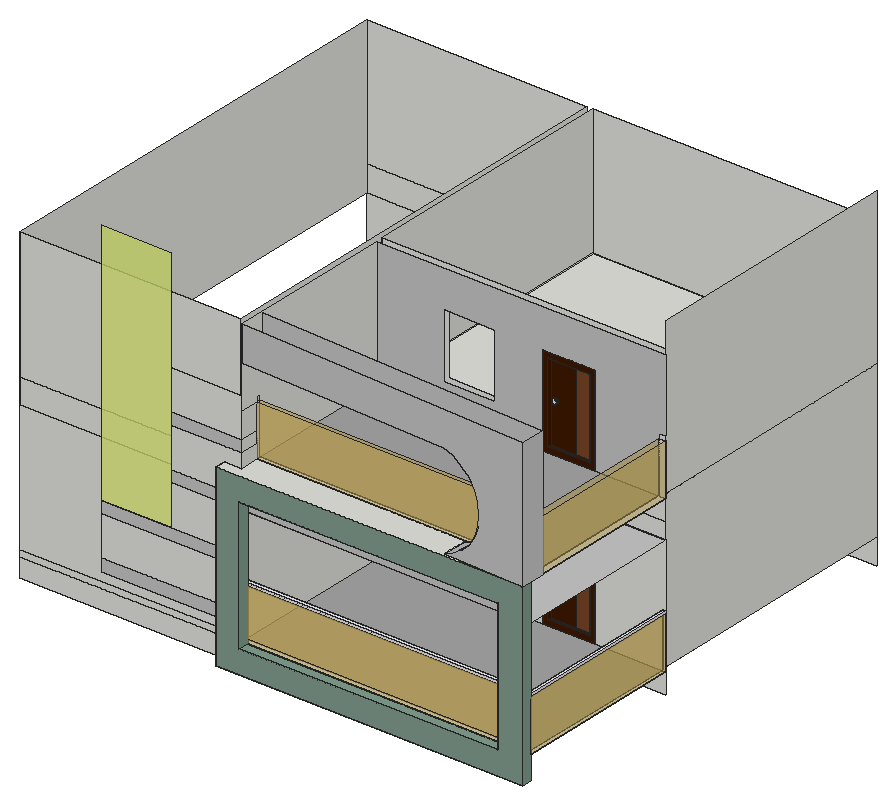
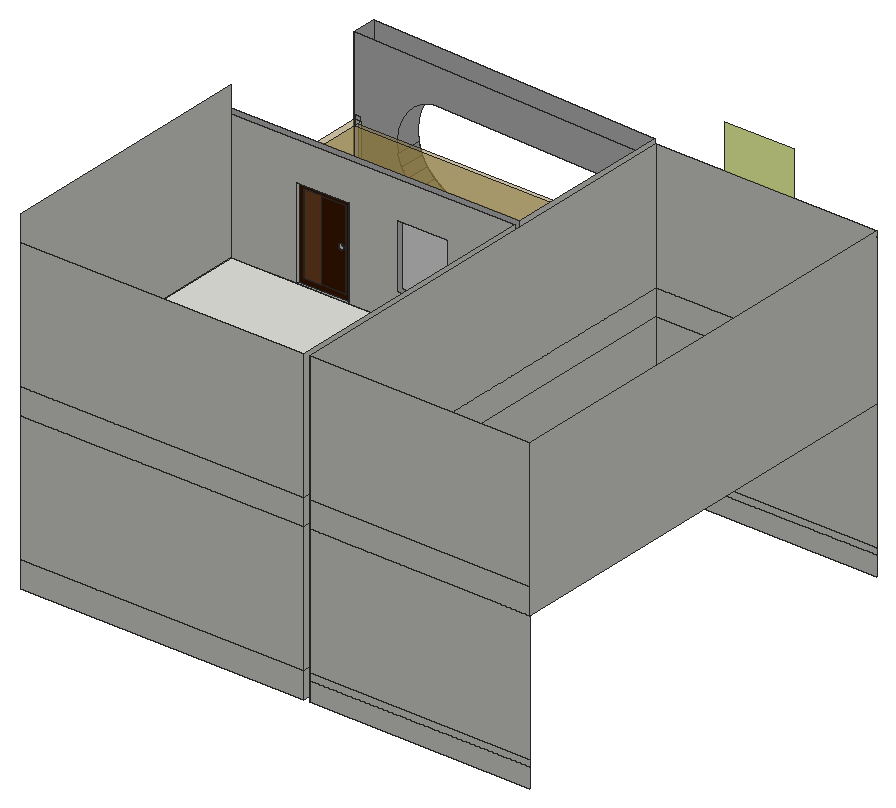
# SketchUp Ruby script. Lengths in inches.
U = 1.inch
M = Sketchup.active_model
def pt(a) = Geom::Point3d.new(a.map { |v| v * U })
def face(e, loops, mat)
  f = e.add_face(loops[0].map { |a| pt(a) })
  loops[1..].each { |l| e.add_face(l.map { |a| pt(a) }).erase! }
  f.material = f.back_material = mat if mat
  f
end
# faces: each face lists its corners as indices into pts; further lists are holes
def faces(e, pts, list, mat = nil) = list.each { |f| face(e, (f[0].is_a?(Array) ? f : [f]).map { |l| l.map { |i| pts[i] } }, mat) }
# xy, xz, yz: faces in a plane at the given z, y or x. An outline is a flat list of corners, or four numbers for a rectangle; further outlines are holes
def ring(l) = l.size == 4 ? [[l[0], l[1]], [l[2], l[1]], [l[2], l[3]], [l[0], l[3]]] : l.each_slice(2).to_a
def flat(e, list, mat, &to3) = list.each { |f| face(e, (f[0].is_a?(Array) ? f : [f]).map { |l| ring(l).map { |u, v| to3.(u, v) } }, mat) }
def xy(e, z, list, mat = nil) = flat(e, list, mat) { |x, y| [x, y, z] }
def xz(e, y, list, mat = nil) = flat(e, list, mat) { |x, z| [x, y, z] }
def yz(e, x, list, mat = nil) = flat(e, list, mat) { |y, z| [x, y, z] }
def lines(e, pts, list) = list.each { |a, b| e.add_line(pt(pts[a]), pt(pts[b])) }
# prism: a flat outline (further loops are holes) pulled along v
def prism(e, loops, v, mat = nil)
  f = face(e, loops, mat); d = Geom::Vector3d.new(v.map { |x| x * U })
  f.pushpull(f.normal.samedirection?(d) ? d.length : -d.length)
end
def box(e, o, s, mat = nil) = prism(e, [[o, [o[0] + s[0], o[1], o[2]], [o[0] + s[0], o[1] + s[1], o[2]], [o[0], o[1] + s[1], o[2]]]], [0, 0, s[2]], mat)
def at(x, y, z, deg = 0) = Geom::Transformation.translation(pt([x, y, z])) * Geom::Transformation.rotation(ORIGIN, Z_AXIS, deg.degrees)
def axes(o, x, y, z) = Geom::Transformation.new([*x, 0, *y, 0, *z, 0, *pt(o).to_a, 1])
def part(name) = M.definitions.add(name)
# library, detail: a bought-in or finely detailed component or shape, given as its bounding box
def library(name, o, s) = part(name).tap { |d| box(d.entities, o, s) }
def detail(e, o, s) = box(e.add_group.entities, o, s)
def put(e, d, t, mat = nil) = e.add_instance(d, t).tap { |i| i.material = mat if mat }
def group(e, t, mat = nil) = e.add_group.tap { |g| g.transformation = t; g.material = mat if mat }.entities
root = M.entities
M.materials.add("[Color B08]").color = [62, 25, 0]
M.materials.add("[Color H08]").color = [130, 158, 143]
M.materials.add("[Color M02]").color = [198, 198, 198]
M.materials.add("[Metal Silver]").color = [234, 233, 238]
M.materials.add("[Stone Vein Gray]").color = [166, 165, 165]
M.materials.add("[Translucent Glass Blue]").color = [201, 149, 0]
M.materials["[Translucent Glass Blue]"].alpha = 0.5
M.materials.add("[Translucent Glass Blue]1").color = [221, 188, 93]
M.materials["[Translucent Glass Blue]1"].alpha = 0.5
M.materials.add("[Translucent Glass Corrugated]").color = [233, 249, 123]
M.materials["[Translucent Glass Corrugated]"].alpha = 0.8
M.materials.add("[Wood Veneer 01]").color = [120, 70, 37]
c1 = part("Group\#1")
xy(c1.entities,0,[[0,0,48,3.5]])
xy(c1.entities,4.73,[[4.73,0,28,3.5],[28,0,43.27,3.5]],"[Color B08]")
xy(c1.entities,79.27,[[4.73,0,28,3.5],[28,0,43.27,3.5]])
xy(c1.entities,84,[[0,0,48,3.5]],"[Color B08]")
xz(c1.entities,0,[[[0,0,48,84],[4.73,4.73,43.27,79.27]]],"[Color B08]")
xz(c1.entities,1.8125,[[8.85,40.5625,9.49,40.61,10.09,40.82,10.62,41.17,11.03,41.66,11.31,42.23,11.43,42.85,11.38,43.49,11.17,44.09,10.82,44.62,10.33,45.03,9.76,45.31,9.14,45.43,8.5,45.38,7.9,45.17,7.375,44.81,6.96,44.33,6.68,43.76,6.5625,43.14,6.61,42.5,6.82,41.9,7.17,41.375,7.66,40.96,8.23,40.68]],"[Metal Silver]")
xz(c1.entities,3.5,[[[0,0,48,84],[4.73,4.73,43.27,79.27]],[[4.73,4.73,28,79.27],[8.85,40.5625,8.23,40.68,7.66,40.96,7.17,41.375,6.82,41.9,6.61,42.5,6.5625,43.14,6.68,43.76,6.96,44.33,7.375,44.81,7.9,45.17,8.5,45.38,9.14,45.43,9.76,45.31,10.33,45.03,10.82,44.62,11.17,44.09,11.38,43.49,11.43,42.85,11.31,42.23,11.03,41.66,10.62,41.17,10.09,40.82,9.49,40.61]]],"[Color B08]")
xz(c1.entities,3.5,[[8.85,40.5625,8.23,40.68,7.66,40.96,7.17,41.375,6.82,41.9,6.61,42.5,6.5625,43.14,6.68,43.76,6.96,44.33,7.375,44.81,7.9,45.17,8.5,45.38,9.14,45.43,9.76,45.31,10.33,45.03,10.82,44.62,11.17,44.09,11.38,43.49,11.43,42.85,11.31,42.23,11.03,41.66,10.62,41.17,10.09,40.82,9.49,40.61]],"[Metal Silver]")
xz(c1.entities,3.5,[[28,4.73,43.27,79.27]],"[Wood Veneer 01]")
yz(c1.entities,0,[[0,0,3.5,84]],"[Color B08]")
yz(c1.entities,4.73,[[0,4.73,3.5,79.27]],"[Color B08]")
yz(c1.entities,43.27,[[0,4.73,3.5,79.27]],"[Color B08]")
yz(c1.entities,48,[[0,0,3.5,84]],"[Color B08]")
p = [[8.23,3.5,40.68],[8.85,3.5,40.5625],[8.85,1.8125,40.5625],[8.23,1.8125,40.68],[9.49,3.5,40.61],[9.49,1.8125,40.61],
  [10.09,3.5,40.82],[10.09,1.8125,40.82],[7.66,3.5,40.96],[7.66,1.8125,40.96],[10.62,3.5,41.17],[10.62,1.8125,41.17],
  [7.17,3.5,41.375],[7.17,1.8125,41.375],[11.03,3.5,41.66],[11.03,1.8125,41.66],[6.82,3.5,41.9],[6.82,1.8125,41.9],
  [11.31,3.5,42.23],[11.31,1.8125,42.23],[6.61,3.5,42.5],[6.61,1.8125,42.5],[11.43,3.5,42.85],[11.43,1.8125,42.85],
  [6.5625,3.5,43.14],[6.5625,1.8125,43.14],[11.38,3.5,43.49],[11.38,1.8125,43.49],[6.68,3.5,43.76],[6.68,1.8125,43.76],
  [11.17,3.5,44.09],[11.17,1.8125,44.09],[6.96,3.5,44.33],[6.96,1.8125,44.33],[10.82,3.5,44.62],[10.82,1.8125,44.62],
  [7.375,3.5,44.81],[7.375,1.8125,44.81],[10.33,3.5,45.03],[10.33,1.8125,45.03],[7.9,3.5,45.17],[7.9,1.8125,45.17],
  [9.76,3.5,45.31],[9.76,1.8125,45.31],[8.5,3.5,45.38],[8.5,1.8125,45.38],[9.14,3.5,45.43],[9.14,1.8125,45.43]]
faces(c1.entities,p,[[0,1,2,3],[1,4,5,2],[4,6,7,5],[8,0,3,9],[6,10,11,7],[12,8,9,13],[10,14,15,11],[16,12,13,17],
  [14,18,19,15],[20,16,17,21],[18,22,23,19],[24,20,21,25],[22,26,27,23],[28,24,25,29],[26,30,31,27],[32,28,29,33],
  [30,34,35,31],[36,32,33,37],[34,38,39,35],[40,36,37,41],[38,42,43,39],[44,40,41,45],[42,46,47,43],[46,44,45,47]],"[Metal Silver]")
c2 = part("Group\#2")
xy(c2.entities,0,[[0,0,48,4.9375]])
xy(c2.entities,3.28,[[23.77,0,25.1875,4.9375]])
xy(c2.entities,3.28,[[3.28,0,23.77,4.9375],[25.1875,0,44.72,4.9375]],"[Color B08]")
xy(c2.entities,56.72,[[23.77,0,25.1875,4.9375]])
xy(c2.entities,56.72,[[3.28,0,23.77,4.9375],[25.1875,0,44.72,4.9375]],"[Color B08]")
xy(c2.entities,60,[[0,0,48,4.9375]],"[Color B08]")
xz(c2.entities,0,[[[0,0,48,60],[3.28,3.28,44.72,56.72]],[23.77,3.28,25.1875,56.72]],"[Color B08]")
xz(c2.entities,4.9375,[[[0,0,48,60],[3.28,3.28,44.72,56.72]],[23.77,3.28,25.1875,56.72]],"[Color B08]")
xz(c2.entities,4.9375,[[3.28,3.28,23.77,56.72],[25.1875,3.28,44.72,56.72]],"[Translucent Glass Blue]")
yz(c2.entities,0,[[0,0,4.9375,60]],"[Color B08]")
yz(c2.entities,3.28,[[0,3.28,4.9375,56.72]],"[Color B08]")
yz(c2.entities,23.77,[[0,3.28,4.9375,56.72]],"[Color B08]")
yz(c2.entities,25.1875,[[0,3.28,4.9375,56.72]],"[Color B08]")
yz(c2.entities,44.72,[[0,3.28,4.9375,56.72]],"[Color B08]")
yz(c2.entities,48,[[0,0,4.9375,60]],"[Color B08]")
xy(root,131.51,[[269.375,132.6875,554.1875,142.1875]],"[Color H08]")
xy(root,153,[[285.75,142.1875,285.75,146.18,550.9,146.18,550.9,299.125,554.1875,299.125,554.1875,142.1875],[285.75,305.125,548.75,550.1875]])
xy(root,153,[[290.875,132.6875,531.17,142.1875]],"[Color H08]")
xy(root,153,[[285.75,146.18,550.9,146.18,550.9,299.125,487.75,299.125,487.75,305.125,439.75,305.125,439.75,299.125,285.75,299.125]],"[Stone Vein Gray]")
xy(root,182.88,[[347.8125,299.125,395.8125,305.125]])
xy(root,201,[[285.75,142.1875,285.75,146.18,550.9,146.18,550.9,299.125,554.1875,299.125,554.1875,142.1875]])
xy(root,203.625,[[285.75,142.1875,554.1875,142.1875,554.1875,299.125,550.9,299.125,550.9,146.18,285.75,146.18]],"[Metal Silver]")
xy(root,237,[[439.75,299.125,487.75,305.125]])
xy(root,242.88,[[347.8125,299.125,395.8125,305.125]])
xy(root,262.5625,[[285.75,142.1875,554.1875,299.125]],"[Color M02]")
xy(root,275.35,[[290.875,132.6875,531.17,142.1875]],"[Color H08]")
xy(root,297,[[269.375,132.6875,554.1875,132.6875,478.91,135.35,479.15,142.1875,479.42,149.6875,479.42,159.75,285.75,159.75,285.75,142.1875,269.375,142.1875],[554.1875,132.6875,554.1875,142.1875,479.15,142.1875,478.91,135.35],[554.1875,132.6875,554.1875,155.45,554.99,155.42],[479.15,142.1875,479.42,149.6875,479.71,158.09,547.7,155.68,554.1875,155.45,554.1875,142.1875],[479.42,149.6875,479.71,158.09,547.7,155.68,547.7,159.75,479.42,159.75],
  [554.1875,155.45,547.7,155.68,547.7,299.125,554.1875,299.125],[285.75,159.75,547.7,163.37],[285.75,305.125,548.75,550.1875]])
xy(root,297,[[285.75,163.37,547.7,163.37,547.7,299.125,487.75,299.125,487.75,305.125,439.75,305.125,439.75,299.125,285.75,299.125]],"[Stone Vein Gray]")
xz(root,132.6875,[[[269.375,131.51,554.1875,297],[290.875,153,531.17,275.35]]],"[Color H08]")
xz(root,142.1875,[[269.375,131.51,554.1875,153],[269.375,153,285.75,165.45],[285.75,153,290.875,201],[531.17,153,554.1875,201],[269.375,165.45,285.75,176.5],
  [155.14,176.5,269.375,213.52],[269.375,176.5,285.75,213.52],[285.75,201,290.875,203.625],[531.17,201,554.1875,203.625],[269.375,213.52,285.75,224.5625],
  [220.2,224.5625,269.375,261.58],[269.375,224.5625,285.75,261.58],[269.375,261.58,285.75,272.625],[531.17,262.5625,554.1875,276.72],[220.2,272.625,269.375,272.625,269.375,297,285.75,297,285.75,309.64,220.2,309.64],
  [220.2,320.6875,285.75,357.7]])
xz(root,142.1875,[[285.75,203.625,290.875,262.5625],[531.17,203.625,554.1875,262.5625]],"[Color H08]")
xz(root,142.1875,[[155.14,165.45,269.375,176.5],[155.14,213.52,269.375,224.5625],[220.2,261.58,269.375,272.625],[290.875,262.5625,531.17,275.35],[220.2,309.64,285.75,320.6875]],"[Color M02]")
xz(root,142.1875,[[290.875,201,531.17,203.625]],"[Metal Silver]")
xz(root,142.1875,[[290.875,153,531.17,201]],"[Translucent Glass Blue]1")
xz(root,142.1875,[[155.14,224.5625,220.2,453.83]],"[Translucent Glass Corrugated]")
xz(root,146.18,[[285.75,201,550.9,203.625]],"[Metal Silver]")
xz(root,146.18,[[285.75,153,550.9,201]],"[Translucent Glass Blue]1")
xz(root,148.1875,[[75,129,279.75,147],[75,147,279.75,153],[75,153,279.75,273],[75,273,279.75,297],[75,297,279.75,417]])
xz(root,159.75,[[285.75,297,547.7,345]],"[Translucent Glass Blue]1")
xz(root,163.37,[[285.75,297,547.7,345]],"[Translucent Glass Blue]1")
xz(root,299.125,[[[285.75,153,439.75,153,439.75,237,487.75,237,487.75,153,550.9,153,550.9,203.625,554.1875,203.625,554.1875,262.5625,285.75,262.5625],[347.8125,182.88,395.8125,242.88]],[550.9,153,554.1875,201],[550.9,201,554.1875,203.625],[547.7,297,554.1875,345]])
xz(root,299.125,[[[285.75,297,439.75,297,439.75,381,487.75,381,487.75,297,547.7,297,547.7,349.125,554.1875,349.125,554.1875,417,285.75,417],[347.4375,322.25,395.4375,382.25]]],"[Color M02]")
xz(root,305.125,[[285.75,129,548.75,153],[[285.75,153,285.75,273,548.75,273,548.75,153,487.75,153,487.75,237,439.75,237,439.75,153],[347.8125,182.88,395.8125,242.88]],[285.75,273,548.75,297],[[285.75,297,285.75,417,548.75,417,548.75,297,487.75,297,487.75,381,439.75,381,439.75,297],[347.4375,322.25,395.4375,382.25]]])
xz(root,550.1875,[[75,129,279.75,147],[285.75,129,548.75,153],[75,147,279.75,153],[75,153,279.75,273],[285.75,153,548.75,273],
  [75,273,279.75,297],[285.75,273,548.75,297],[75,297,279.75,417],[285.75,297,548.75,417]])
yz(root,75,[[148.1875,273,550.1875,417]])
yz(root,269.375,[[132.6875,131.51,142.1875,297]],"[Color H08]")
yz(root,279.75,[[148.1875,129,550.1875,147],[148.1875,147,211.54,153],[211.54,147,221.6,153],[221.6,147,550.1875,153],[148.1875,153,550.1875,273],
  [148.1875,273,550.1875,297],[148.1875,297,550.1875,417]])
yz(root,285.75,[[305.125,129,550.1875,153],[142.1875,153,146.18,201],[146.18,153,299.125,153,299.125,262.5625,142.1875,262.5625,142.1875,203.625,146.18,203.625],[305.125,153,550.1875,273],[142.1875,201,146.18,203.625],
  [305.125,273,550.1875,297],[142.1875,297,159.75,309.64],[163.37,297,299.125,297,299.125,417,142.1875,417,142.1875,345,159.75,345,159.75,349.125,163.37,349.125],[159.75,297,163.37,345],[305.125,297,550.1875,417],
  [142.1875,309.64,159.75,320.6875],[142.1875,320.6875,159.75,345]])
yz(root,290.875,[[132.6875,153,142.1875,275.35]],"[Color H08]")
yz(root,347.8125,[[299.125,182.88,305.125,242.88]])
yz(root,395.8125,[[299.125,182.88,305.125,242.88]])
yz(root,439.75,[[299.125,153,305.125,237],[299.125,297,305.125,381]])
yz(root,487.75,[[299.125,153,305.125,237],[299.125,297,305.125,381]])
yz(root,531.17,[[132.6875,153,142.1875,275.35]])
yz(root,547.7,[[155.68,297,159.75,345],[159.75,297,163.37,345]])
yz(root,547.7,[[163.37,297,299.125,345]],"[Translucent Glass Blue]1")
yz(root,548.75,[[305.125,153,550.1875,297],[305.125,297,550.1875,441]])
yz(root,550.9,[[146.18,201,299.125,203.625]],"[Metal Silver]")
yz(root,550.9,[[146.18,153,299.125,201]],"[Translucent Glass Blue]1")
yz(root,554.1875,[[132.6875,131.51,142.1875,297]],"[Color H08]")
yz(root,554.1875,[[142.1875,201,299.125,203.625]],"[Metal Silver]")
yz(root,554.1875,[[142.1875,153,299.125,201],[155.45,297,299.125,345]],"[Translucent Glass Blue]1")
p = [[285.75,142.1875,384.9],[478.91,135.35,384.9],[488.11,135.03,381.29],[496.32,134.74,375.78],[503.15,134.49,368.62],[508.27,134.3125,360.15],
  [511.4375,134.2,350.78],[512.51,134.16,340.95],[511.4375,134.2,331.12],[508.27,134.3125,321.74],[503.15,134.49,313.28],[496.32,134.74,306.125],
  [488.11,135.03,300.61],[478.91,135.35,297],[554.1875,132.6875,297],[554.1875,132.6875,417],[285.75,142.1875,417],[285.75,142.1875,416.8125],
  [285.75,142.1875,405.77],[554.99,155.42,297],[554.99,155.42,417],[488.92,157.76,300.61],[479.71,158.09,297],[479.42,149.6875,297],
  [479.15,142.1875,297],[479.71,158.09,384.9],[286.55,164.92,384.9],[286.55,164.92,417],[554.1875,155.45,417],[554.1875,155.45,297],
  [554.1875,155.45,345],[554.1875,155.45,349.125],[547.7,155.68,349.125],[547.7,155.68,345],[547.7,155.68,297],[497.125,157.47,306.125],
  [503.95,157.23,313.28],[509.07,157.05,321.74],[512.24,156.9375,331.12],[513.32,156.9,340.95],[512.24,156.9375,350.78],[509.07,157.05,360.15],
  [503.95,157.23,368.62],[497.125,157.47,375.78],[488.92,157.76,381.29]]
faces(root,p,[[0,1,2,3,4,5,6,7,8,9,10,11,12,13,14,15,16,17,18],[14,19,20,15],[12,21,22,23,24,13],[25,26,27,28,20,19,29,30,31,32,33,34,22,21,35,36,37,38,39,40,41,42,43,44],[11,35,21,12],[10,36,35,11],[9,37,36,10],[8,38,37,9]],"[Color M02]")
faces(root,p,[[29,34,33,30]])
put(root,c1,at(439.75,299.125,153))
put(root,c2,at(347.8125,299.125,182.88))
put(root,c1,at(439.75,299.125,297))
